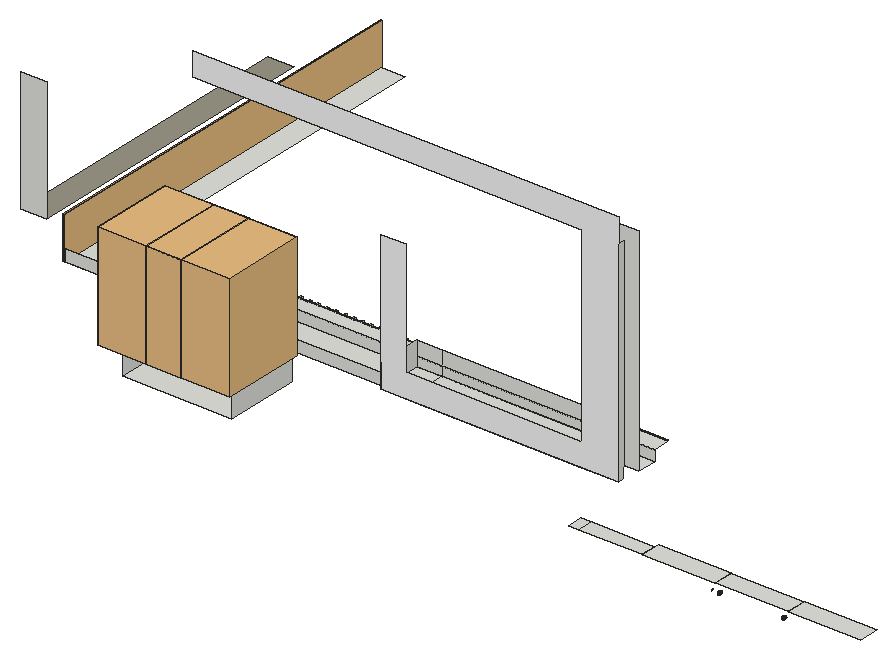
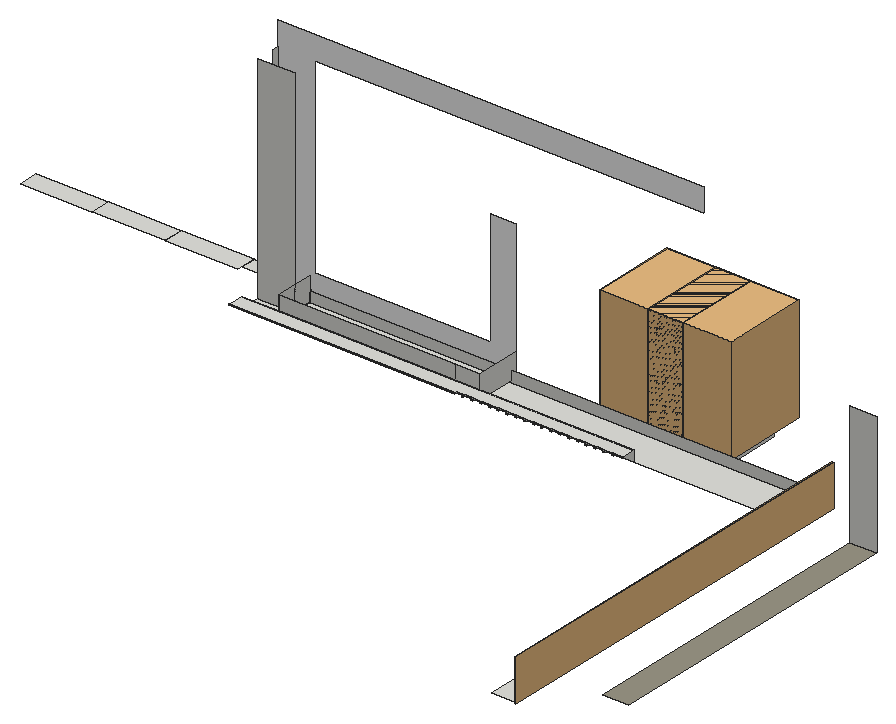
# SketchUp Ruby script. Lengths in inches.
U = 1.inch
M = Sketchup.active_model
def pt(a) = Geom::Point3d.new(a.map { |v| v * U })
def face(e, loops, mat)
  f = e.add_face(loops[0].map { |a| pt(a) })
  loops[1..].each { |l| e.add_face(l.map { |a| pt(a) }).erase! }
  f.material = f.back_material = mat if mat
  f
end
# faces: each face lists its corners as indices into pts; further lists are holes
def faces(e, pts, list, mat = nil) = list.each { |f| face(e, (f[0].is_a?(Array) ? f : [f]).map { |l| l.map { |i| pts[i] } }, mat) }
# xy, xz, yz: faces in a plane at the given z, y or x. An outline is a flat list of corners, or four numbers for a rectangle; further outlines are holes
def ring(l) = l.size == 4 ? [[l[0], l[1]], [l[2], l[1]], [l[2], l[3]], [l[0], l[3]]] : l.each_slice(2).to_a
def flat(e, list, mat, &to3) = list.each { |f| face(e, (f[0].is_a?(Array) ? f : [f]).map { |l| ring(l).map { |u, v| to3.(u, v) } }, mat) }
def xy(e, z, list, mat = nil) = flat(e, list, mat) { |x, y| [x, y, z] }
def xz(e, y, list, mat = nil) = flat(e, list, mat) { |x, z| [x, y, z] }
def yz(e, x, list, mat = nil) = flat(e, list, mat) { |y, z| [x, y, z] }
def lines(e, pts, list) = list.each { |a, b| e.add_line(pt(pts[a]), pt(pts[b])) }
# prism: a flat outline (further loops are holes) pulled along v
def prism(e, loops, v, mat = nil)
  f = face(e, loops, mat); d = Geom::Vector3d.new(v.map { |x| x * U })
  f.pushpull(f.normal.samedirection?(d) ? d.length : -d.length)
end
def box(e, o, s, mat = nil) = prism(e, [[o, [o[0] + s[0], o[1], o[2]], [o[0] + s[0], o[1] + s[1], o[2]], [o[0], o[1] + s[1], o[2]]]], [0, 0, s[2]], mat)
def at(x, y, z, deg = 0) = Geom::Transformation.translation(pt([x, y, z])) * Geom::Transformation.rotation(ORIGIN, Z_AXIS, deg.degrees)
def axes(o, x, y, z) = Geom::Transformation.new([*x, 0, *y, 0, *z, 0, *pt(o).to_a, 1])
def part(name) = M.definitions.add(name)
# library, detail: a bought-in or finely detailed component or shape, given as its bounding box
def library(name, o, s) = part(name).tap { |d| box(d.entities, o, s) }
def detail(e, o, s) = box(e.add_group.entities, o, s)
def put(e, d, t, mat = nil) = e.add_instance(d, t).tap { |i| i.material = mat if mat }
def group(e, t, mat = nil) = e.add_group.tap { |g| g.transformation = t; g.material = mat if mat }.entities
root = M.entities
M.materials.add("[0129_WhiteSmoke]1").color = [245, 245, 245]
M.materials.add("[Concrete Tile]").color = [155, 150, 134]
c1 = library("plant (1)",[-35.72,-28.42,0],[66.31,67.39,84.38])
c2 = part("glass-railing")
detail(c2.entities,[0,0,0],[1.26,75.59,33.1875])
xy(root,138.0625,[[2608.61,801.78,2617.01,814.22],[2617.01,801.78,2666.66,814.22],[2667.6,801.78,2724.71,817.6],[2725.77,801.78,2782.76,817.6],[2784.08,801.78,2840.8125,817.6]])
xy(root,138.1875,[[2273.89,776.37,2360.78,836.7]])
xy(root,153.5625,[[2170.98,846.1,2587.8,846.1,2587.8,861.24,2617.01,861.24,2617.01,877.14,2191.39,877.14,2191.39,1160.85,2170.98,1160.85]])
xy(root,154.75,[[2427.73,840.97,2447.38,877.14],[2447.38,840.97,2587.8,877.14],[2587.8,840.97,2617.01,845.35]])
xy(root,156.5,[[2112.0625,877.14,2132.8125,1122.97]],"[Concrete Tile]")
xy(root,162.125,[[2305.05,877.14,2305.05,888.95,2310.46,888.95,2310.46,890.39,2312.11,890.39,2312.11,888.95,2317.52,888.95,2317.52,890.39,2319.11,890.39,2319.11,888.95,2324.52,888.95,2324.52,890.39,2326.11,890.39,2326.11,888.95,2331.52,888.95,2331.52,890.39,2333.11,890.39,2333.11,888.95,2338.52,888.95,2338.52,890.39,2340.11,890.39,2340.11,888.95,2345.52,888.95,2345.52,890.39,2347.11,890.39,2347.11,888.95,2352.52,888.95,2352.52,890.39,2354.11,890.39,2354.11,888.95,2359.52,888.95,2359.52,890.39,2361.11,890.39,2361.11,888.95,2366.52,888.95,2366.52,890.39,2368.11,890.39,2368.11,888.95,2373.52,888.95,2373.52,890.39,2375.11,890.39,2375.11,888.95,2380.52,888.95,2380.52,890.39,2382.11,890.39,2382.11,888.95,2387.52,888.95,2387.52,890.39,2389.11,890.39,2389.11,888.95,2394.52,888.95,2394.52,890.39,2396.11,890.39,2396.11,888.83,2401.52,888.83,2401.52,890.39,2403.11,890.39,2403.11,888.83,2408.52,888.83,2408.52,890.39,2410.11,890.39,2410.11,888.83,2415.52,888.83,2415.52,890.39,2417.11,890.39,2417.11,888.83,2422.52,888.83,2422.52,890.39,2424.11,890.39,2424.11,888.83,2429.52,888.83,2429.52,890.39,2431.11,890.39,2431.11,888.83,2436.52,888.83,2436.52,890.39,2617.01,890.39,2617.01,877.14]])
xz(root,836.7,[[2273.89,138.1875,2360.78,183.3125]])
xz(root,840.97,[[2427.73,154.75,2617.01,154.75,2617.01,343.4375,2278.36,343.4375,2278.36,324.5625,2587.8,324.5625,2587.8,173.4375,2447.38,173.4375,2447.38,264.75,2427.73,264.75]],"[0129_WhiteSmoke]1")
xz(root,845.35,[[2587.8,154.75,2617.01,163]])
xz(root,846.1,[[2170.98,153.5625,2587.8,162.75]])
xz(root,861.24,[[2587.8,153.5625,2617.01,324.5625]])
xz(root,877.14,[[2305.05,153.5625,2617.01,153.5625,2617.01,162.125,2587.8,162.125,2587.8,154.75,2427.73,154.75,2427.73,162.125,2305.05,162.125],[2427.73,154.75,2447.38,162.125],[2447.38,154.75,2587.8,162.125],[2112.0625,156.5,2132.8125,254.125],[2427.73,162.125,2447.38,173.4375],
  [2447.38,162.125,2587.8,173.4375]])
xz(root,888.83,[[2396.11,162.125,2401.52,162.75],[2403.11,162.125,2408.52,162.75],[2410.11,162.125,2415.52,162.75],[2417.11,162.125,2422.52,162.75],[2424.11,162.125,2429.52,162.75],
  [2431.11,162.125,2436.52,162.75]])
xz(root,888.95,[[2305.05,162.125,2310.46,162.75],[2312.11,162.125,2317.52,162.75],[2319.11,162.125,2324.52,162.75],[2326.11,162.125,2331.52,162.75],[2333.11,162.125,2338.52,162.75],
  [2340.11,162.125,2345.52,162.75],[2347.11,162.125,2352.52,162.75],[2354.11,162.125,2359.52,162.75],[2361.11,162.125,2366.52,162.75],[2368.11,162.125,2373.52,162.75],
  [2375.11,162.125,2380.52,162.75],[2382.11,162.125,2387.52,162.75],[2389.11,162.125,2394.52,162.75]])
xz(root,890.39,[[2310.46,162.125,2312.11,162.75],[2317.52,162.125,2319.11,162.75],[2324.52,162.125,2326.11,162.75],[2331.52,162.125,2333.11,162.75],[2338.52,162.125,2340.11,162.75],
  [2345.52,162.125,2347.11,162.75],[2352.52,162.125,2354.11,162.75],[2359.52,162.125,2361.11,162.75],[2366.52,162.125,2368.11,162.75],[2373.52,162.125,2375.11,162.75],
  [2380.52,162.125,2382.11,162.75],[2387.52,162.125,2389.11,162.75],[2394.52,162.125,2396.11,162.75],[2401.52,162.125,2403.11,162.75],[2408.52,162.125,2410.11,162.75],
  [2415.52,162.125,2417.11,162.75],[2422.52,162.125,2424.11,162.75],[2429.52,162.125,2431.11,162.75],[2436.52,162.125,2439.65,162.75],[2439.65,162.125,2617.01,162.75]])
yz(root,2273.89,[[776.37,138.1875,836.7,183.3125]])
yz(root,2310.46,[[888.95,162.125,890.39,162.75]])
yz(root,2312.11,[[888.95,162.125,890.39,162.75]])
yz(root,2317.52,[[888.95,162.125,890.39,162.75]])
yz(root,2319.11,[[888.95,162.125,890.39,162.75]])
yz(root,2324.52,[[888.95,162.125,890.39,162.75]])
yz(root,2326.11,[[888.95,162.125,890.39,162.75]])
yz(root,2331.52,[[888.95,162.125,890.39,162.75]])
yz(root,2333.11,[[888.95,162.125,890.39,162.75]])
yz(root,2338.52,[[888.95,162.125,890.39,162.75]])
yz(root,2340.11,[[888.95,162.125,890.39,162.75]])
yz(root,2345.52,[[888.95,162.125,890.39,162.75]])
yz(root,2347.11,[[888.95,162.125,890.39,162.75]])
yz(root,2352.52,[[888.95,162.125,890.39,162.75]])
yz(root,2354.11,[[888.95,162.125,890.39,162.75]])
yz(root,2359.52,[[888.95,162.125,890.39,162.75]])
yz(root,2360.78,[[776.37,138.1875,836.7,183.3125]])
yz(root,2361.11,[[888.95,162.125,890.39,162.75]])
yz(root,2366.52,[[888.95,162.125,890.39,162.75]])
yz(root,2368.11,[[888.95,162.125,890.39,162.75]])
yz(root,2373.52,[[888.95,162.125,890.39,162.75]])
yz(root,2375.11,[[888.95,162.125,890.39,162.75]])
yz(root,2380.52,[[888.95,162.125,890.39,162.75]])
yz(root,2382.11,[[888.95,162.125,890.39,162.75]])
yz(root,2387.52,[[888.95,162.125,890.39,162.75]])
yz(root,2389.11,[[888.95,162.125,890.39,162.75]])
yz(root,2394.52,[[888.95,162.125,890.39,162.75]])
yz(root,2396.11,[[888.83,162.125,890.39,162.75]])
yz(root,2401.52,[[888.83,162.125,890.39,162.75]])
yz(root,2403.11,[[888.83,162.125,890.39,162.75]])
yz(root,2408.52,[[888.83,162.125,890.39,162.75]])
yz(root,2410.11,[[888.83,162.125,890.39,162.75]])
yz(root,2415.52,[[888.83,162.125,890.39,162.75]])
yz(root,2417.11,[[888.83,162.125,890.39,162.75]])
yz(root,2422.52,[[888.83,162.125,890.39,162.75]])
yz(root,2424.11,[[888.83,162.125,890.39,162.75]])
yz(root,2427.73,[[840.97,154.75,877.14,173.4375]])
yz(root,2429.52,[[888.83,162.125,890.39,162.75]])
yz(root,2431.11,[[888.83,162.125,890.39,162.75]])
yz(root,2436.52,[[888.83,162.125,890.39,162.75]])
yz(root,2587.8,[[846.1,153.5625,861.24,154.75],[845.35,154.75,846.1,162.75],[846.1,154.75,861.24,173.4375],[861.24,154.75,877.14,173.4375]])
yz(root,2617.01,[[840.97,154.75,845.35,154.75,845.35,163,846.1,163,846.1,324.5625,840.97,324.5625]])
p = [[2729.1,801.78,132.03],[2729.37,801.78,131.92],[2729.37,799.91,131.92],[2729.1,799.91,132.03],[2729.66,801.78,131.88],[2729.66,799.91,131.88],
  [2729.95,801.78,131.92],[2729.95,799.91,131.92],[2730.22,801.78,132.03],[2730.22,799.91,132.03],[2780.22,801.78,132.03],[2780.49,801.78,131.92],
  [2780.49,799.91,131.92],[2780.22,799.91,132.03],[2780.79,801.78,131.88],[2780.79,799.91,131.88],[2781.08,801.78,131.92],[2781.08,799.91,131.92],
  [2781.35,801.78,132.03],[2781.35,799.91,132.03],[2728.86,801.78,132.21],[2728.86,799.91,132.21],[2730.46,801.78,132.21],[2730.46,799.91,132.21],
  [2779.99,801.78,132.21],[2779.99,799.91,132.21],[2781.58,801.78,132.21],[2781.58,799.91,132.21],[2728.6875,801.78,132.44],[2728.6875,799.91,132.44],
  [2730.63,801.78,132.44],[2730.63,799.91,132.44],[2779.8125,801.78,132.44],[2779.8125,799.91,132.44],[2781.76,801.78,132.44],[2781.76,799.91,132.44],
  [2728.57,801.78,132.71],[2728.57,799.91,132.71],[2730.75,801.78,132.71],[2730.75,799.91,132.71],[2779.7,801.78,132.71],[2779.7,799.91,132.71],
  [2781.87,801.78,132.71],[2781.87,799.91,132.71],[2723.7,801.78,132.71],[2723.73,801.78,133],[2723.73,799.91,133],[2723.7,799.91,132.71],
  [2728.54,801.78,133],[2728.54,799.91,133],[2730.79,801.78,133],[2730.79,799.91,133],[2779.66,801.78,133],[2779.66,799.91,133],
  [2781.91,801.78,133],[2781.91,799.91,133],[2723.7,801.78,133.29],[2723.7,799.91,133.29],[2728.57,801.78,133.29],[2728.57,799.91,133.29],
  [2730.75,801.78,133.29],[2730.75,799.91,133.29],[2779.7,801.78,133.29],[2779.7,799.91,133.29],[2781.87,801.78,133.29],[2781.87,799.91,133.29],
  [2728.6875,801.78,133.57],[2728.6875,799.91,133.57],[2730.63,801.78,133.57],[2730.63,799.91,133.57],[2779.8125,801.78,133.57],[2779.8125,799.91,133.57],
  [2781.76,801.78,133.57],[2781.76,799.91,133.57],[2728.86,801.78,133.8],[2728.86,799.91,133.8],[2730.46,801.78,133.8],[2730.46,799.91,133.8],
  [2779.99,801.78,133.8],[2779.99,799.91,133.8],[2781.58,801.78,133.8],[2781.58,799.91,133.8],[2729.1,801.78,133.98],[2729.1,799.91,133.98],
  [2730.22,801.78,133.98],[2730.22,799.91,133.98],[2780.22,801.78,133.98],[2780.22,799.91,133.98],[2781.35,801.78,133.98],[2781.35,799.91,133.98],
  [2729.37,801.78,134.09],[2729.37,799.91,134.09],[2729.95,801.78,134.09],[2729.95,799.91,134.09],[2780.49,801.78,134.09],[2780.49,799.91,134.09],
  [2781.08,801.78,134.09],[2781.08,799.91,134.09],[2729.66,801.78,134.13],[2729.66,799.91,134.13],[2780.79,801.78,134.13],[2780.79,799.91,134.13]]
faces(root,p,[[0,1,2,3],[1,4,5,2],[4,6,7,5],[6,8,9,7],[10,11,12,13],[11,14,15,12],[14,16,17,15],[16,18,19,17],
  [20,0,3,21],[8,22,23,9],[24,10,13,25],[18,26,27,19],[28,20,21,29],[22,30,31,23],[32,24,25,33],[26,34,35,27],
  [36,28,29,37],[30,38,39,31],[40,32,33,41],[34,42,43,35],[44,45,46,47],[48,36,37,49],[38,50,51,39],[52,40,41,53],
  [42,54,55,43],[45,56,57,46],[58,48,49,59],[50,60,61,51],[62,52,53,63],[54,64,65,55],[66,58,59,67],[60,68,69,61],
  [70,62,63,71],[64,72,73,65],[74,66,67,75],[68,76,77,69],[78,70,71,79],[72,80,81,73],[82,74,75,83],[76,84,85,77],
  [86,78,79,87],[80,88,89,81],[90,82,83,91],[84,92,93,85],[94,86,87,95],[88,96,97,89],[98,90,91,99],[92,98,99,93],
  [100,94,95,101],[96,100,101,97]])
put(root,c1,at(2292.9,800.97,155.86))
put(root,c1,at(2331.47,800.97,155.86))
put(root,c2,axes([2170.98,846.1,153.5625],[1,0,0],[0,4.1738,0],[0,0,1]))
